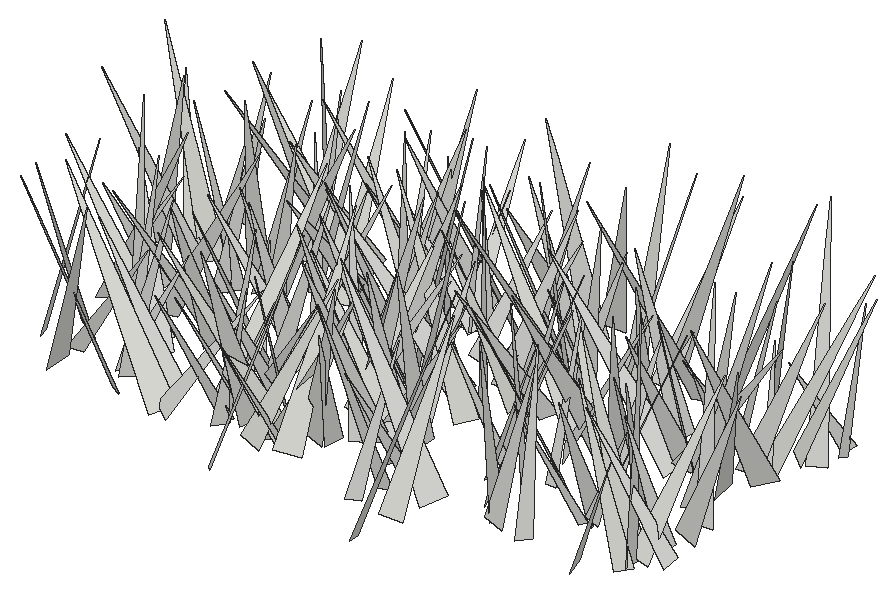
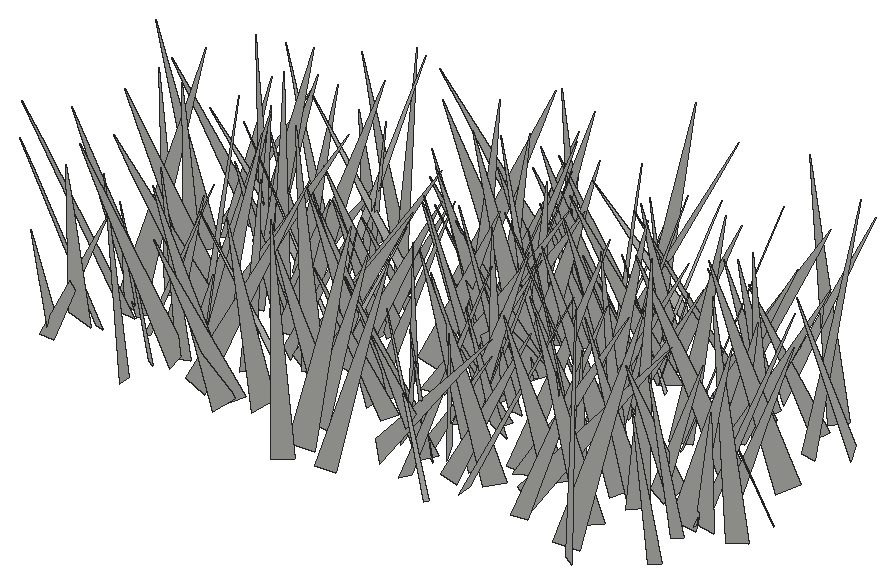
# SketchUp Ruby script. Lengths in inches.
U = 1.inch
M = Sketchup.active_model
def pt(a) = Geom::Point3d.new(a.map { |v| v * U })
def face(e, loops, mat)
  f = e.add_face(loops[0].map { |a| pt(a) })
  loops[1..].each { |l| e.add_face(l.map { |a| pt(a) }).erase! }
  f.material = f.back_material = mat if mat
  f
end
# faces: each face lists its corners as indices into pts; further lists are holes
def faces(e, pts, list, mat = nil) = list.each { |f| face(e, (f[0].is_a?(Array) ? f : [f]).map { |l| l.map { |i| pts[i] } }, mat) }
# xy, xz, yz: faces in a plane at the given z, y or x. An outline is a flat list of corners, or four numbers for a rectangle; further outlines are holes
def ring(l) = l.size == 4 ? [[l[0], l[1]], [l[2], l[1]], [l[2], l[3]], [l[0], l[3]]] : l.each_slice(2).to_a
def flat(e, list, mat, &to3) = list.each { |f| face(e, (f[0].is_a?(Array) ? f : [f]).map { |l| ring(l).map { |u, v| to3.(u, v) } }, mat) }
def xy(e, z, list, mat = nil) = flat(e, list, mat) { |x, y| [x, y, z] }
def xz(e, y, list, mat = nil) = flat(e, list, mat) { |x, z| [x, y, z] }
def yz(e, x, list, mat = nil) = flat(e, list, mat) { |y, z| [x, y, z] }
def lines(e, pts, list) = list.each { |a, b| e.add_line(pt(pts[a]), pt(pts[b])) }
# prism: a flat outline (further loops are holes) pulled along v
def prism(e, loops, v, mat = nil)
  f = face(e, loops, mat); d = Geom::Vector3d.new(v.map { |x| x * U })
  f.pushpull(f.normal.samedirection?(d) ? d.length : -d.length)
end
def box(e, o, s, mat = nil) = prism(e, [[o, [o[0] + s[0], o[1], o[2]], [o[0] + s[0], o[1] + s[1], o[2]], [o[0], o[1] + s[1], o[2]]]], [0, 0, s[2]], mat)
def at(x, y, z, deg = 0) = Geom::Transformation.translation(pt([x, y, z])) * Geom::Transformation.rotation(ORIGIN, Z_AXIS, deg.degrees)
def axes(o, x, y, z) = Geom::Transformation.new([*x, 0, *y, 0, *z, 0, *pt(o).to_a, 1])
def part(name) = M.definitions.add(name)
# library, detail: a bought-in or finely detailed component or shape, given as its bounding box
def library(name, o, s) = part(name).tap { |d| box(d.entities, o, s) }
def detail(e, o, s) = box(e.add_group.entities, o, s)
def put(e, d, t, mat = nil) = e.add_instance(d, t).tap { |i| i.material = mat if mat }
def group(e, t, mat = nil) = e.add_group.tap { |g| g.transformation = t; g.material = mat if mat }.entities
root = M.entities
c1 = part("fur_instance\#9")
p = [[0.8125,0,1.79],[0.67,-0.02,1.48],[0,-0.11,0],[0,0.11,0]]
faces(c1.entities,p,[[0,1,2,3]])
put(root,c1,axes([504.42,389.3125,-21.66],[8.18505,-1.50624,0.16494],[-1.43272,-7.98824,-1.85106],[-0.49323,-1.79175,8.11402]))
put(root,c1,axes([531.82,383.56,-21.66],[7.42778,3.7642,0.92799],[3.25227,-7.14156,2.93652],[-2.11023,2.24305,7.79217]))
put(root,c1,axes([521.25,389.9,-21.66],[-3.70308,-3.24105,0.05421],[-3.08159,3.54543,1.46762],[1.00557,-1.07036,4.69716]))
put(root,c1,axes([518.14,391.06,-21.66],[6.29678,-5.28708,1.00032],[-4.88133,-6.26054,-2.36253],[-2.26416,-1.20654,7.87535]))
put(root,c1,axes([509.29,388.8125,-21.66],[-4.9129,-5.75828,0.52895],[-5.68371,4.68095,-1.83254],[-1.06438,1.58274,7.34412]))
put(root,c1,axes([544.375,389.15,-21.66],[5.4983,0.81734,0.21266],[0.84397,-5.26527,-1.58403],[0.03145,-1.59793,5.32824]))
put(root,c1,axes([520.83,390.58,-21.66],[-8.10416,-1.22815,0.06312],[-1.16757,7.81624,2.17553],[0.38615,-2.14192,7.90272]))
put(root,c1,axes([516.7,390.24,-21.66],[0.11807,-5.18176,0.38422],[-4.95689,-0.22756,-1.54584],[-1.55804,0.33133,4.94722]))
put(root,c1,axes([529.51,389.47,-21.66],[-1.62801,-6.13851,1.48062],[-6.15059,1.19536,-1.80699],[-1.42958,1.84764,6.08822]))
put(root,c1,axes([517.17,391.55,-21.66],[-4.17954,-4.03403,0.06779],[-3.83281,4.00041,1.74723],[1.26,-1.21235,5.53978]))
put(root,c1,axes([532,386.88,-21.66],[-2.25135,6.36064,1.32657],[6.19225,2.52565,-1.60099],[1.96812,-0.67041,6.55463]))
put(root,c1,axes([519.65,384.83,-21.66],[5.70548,5.18554,0.14342],[4.71826,-5.27598,3.06024],[-2.15603,2.1765,7.07653]))
put(root,c1,axes([528.83,387.26,-21.66],[-4.17558,2.72173,1.55923],[2.19552,4.39009,-1.78362],[2.24025,0.77057,4.65424]))
put(root,c1,axes([522.16,391.57,-21.66],[0.1957,-7.90399,1.09327],[-7.43409,0.21668,2.89722],[2.89871,1.0893,7.35646]))
put(root,c1,axes([512.96,388.73,-21.66],[-5.23637,6.32875,0.17784],[5.87309,4.76933,3.20385],[-2.36465,-2.16904,7.5636]))
put(root,c1,axes([513.02,388.52,-21.66],[2.725,5.40327,0.30402],[4.86473,-2.29653,-2.78814],[2.3711,-1.498,5.37096]))
put(root,c1,axes([532.75,390.09,-21.66],[-7.09229,4.18803,1.11711],[4.32642,6.70959,2.31334],[-0.26383,-2.55536,7.90497]))
put(root,c1,axes([536.72,391.13,-21.66],[6.67439,0.3641,2.55328],[0.99441,-6.8993,-1.61558],[-2.3797,-1.86182,6.48614]))
put(root,c1,axes([537.26,390.22,-21.66],[0.1838,-6.38239,2.38865],[-6.46729,0.58989,2.0738],[2.14821,2.32195,6.03888]))
put(root,c1,axes([516.36,390.43,-21.66],[-1.2496,-4.95098,2.04852],[-4.91628,1.89585,1.58307],[2.13046,1.47094,4.85465]))
put(root,c1,axes([519.625,388.79,-21.66],[0.86928,6.52033,1.58307],[6.24969,-0.2059,-2.58369],[2.44176,-1.79425,6.04937]))
put(root,c1,axes([529.21,391.82,-21.66],[1.40326,-4.201,0.43994],[-3.89786,-1.46649,-1.57071],[-1.62745,-0.10993,4.1413]))
put(root,c1,axes([523.49,392.05,-21.66],[4.86782,-2.47433,0.4659],[-2.27673,-4.75873,-1.48527],[-1.07512,-1.1257,5.25471]))
put(root,c1,axes([503.3,393.65,-21.66],[-3.16063,-7.46069,0.64697],[-7.21635,3.22195,1.90087],[2.00118,-0.16476,7.87643]))
put(root,c1,axes([518.74,393.38,-21.66],[-3.46675,-5.54657,1.13696],[-5.08588,3.63649,2.23277],[2.48816,-0.29493,6.14797]))
put(root,c1,axes([511.83,391.42,-21.66],[-4.61226,3.61546,0.79034],[3.61757,4.1381,2.18138],[-0.78062,-2.18488,5.43931]))
put(root,c1,axes([516.79,389.37,-21.66],[-5.68198,1.58826,2.45655],[1.00817,6.10119,-1.61279],[2.74605,1.04639,5.67506]))
put(root,c1,axes([525.66,393.66,-21.66],[3.52912,-6.81057,1.30534],[-6.45742,-3.76145,-2.16695],[-2.52774,0.10047,7.35818]))
put(root,c1,axes([546.97,390.64,-21.66],[-2.40654,5.51072,1.54274],[5.60544,1.9331,1.83892],[-1.15197,-2.10585,5.72519]))
put(root,c1,axes([517.65,394.1,-21.66],[-5.63617,-2.55407,1.20627],[-1.85262,5.37498,2.72438],[2.13217,-2.08115,5.55585]))
put(root,c1,axes([520.44,390.14,-21.66],[6.21247,-1.9108,0.54363],[-1.98453,-5.88708,1.9863],[0.09123,2.05733,6.18874]))
put(root,c1,axes([504.27,391.19,-21.66],[3.95823,-3.37287,0.12226],[-3.1364,-3.60629,2.0534],[1.24667,1.63622,4.7778]))
put(root,c1,axes([539.9,389.82,-21.66],[-5.67085,1.89535,1.35099],[1.57668,5.74544,-1.44226],[1.71219,0.98676,5.80265]))
put(root,c1,axes([507.76,391.4,-21.66],[2.74788,4.31889,0.7575],[4.17328,-2.30167,-2.01583],[1.34551,-1.68135,4.70533]))
put(root,c1,axes([522.2,389.19,-21.66],[-3.86216,7.0455,1.20437],[6.7899,4.04407,-1.88376],[2.2331,-0.11104,7.81068]))
put(root,c1,axes([548.68,393.02,-21.66],[-5.67147,0.82087,0.04901],[0.80443,5.46726,1.5178],[-0.17066,-1.50898,5.5259]))
put(root,c1,axes([508.2,391.07,-21.66],[5.34451,-1.51745,2.02584],[-2.07356,-5.33917,1.4711],[-1.45157,2.03988,5.35746]))
put(root,c1,axes([520.91,391.54,-21.66],[0.51844,5.23573,1.343],[5.13497,-0.0558,-1.76472],[1.68777,-1.43851,4.95655]))
put(root,c1,axes([516.24,391.59,-21.66],[-4.21104,-1.2398,0.43934],[-1.31531,3.95873,-1.43574],[-0.00925,1.50143,4.14832]))
put(root,c1,axes([541.25,395.02,-21.66],[5.27025,-2.47106,0.85487],[-2.00329,-5.05203,-2.25305],[-1.68041,-1.72721,5.36707]))
put(root,c1,axes([514.88,392.86,-21.66],[3.85978,2.30102,0.3483],[2.28006,-3.60384,-1.45862],[0.46617,-1.42533,4.2503]))
put(root,c1,axes([547.47,394.24,-21.66],[-4.78026,1.17069,2.19317],[1.89155,4.79719,1.56216],[1.61324,-2.15588,4.66702]))
put(root,c1,axes([545.3,393.41,-21.66],[3.76435,-5.16952,3.38659],[-5.24976,-4.76711,-1.44149],[-3.26082,1.70703,6.23028]))
put(root,c1,axes([508.73,390.62,-21.66],[-6.51752,1.2418,2.00991],[0.54856,6.53189,-2.25684],[2.29801,1.9627,6.23913]))
put(root,c1,axes([509.04,393.28,-21.66],[-3.24563,2.42896,0.17461],[2.25293,2.88449,1.75171],[-0.92447,-1.49811,3.65588]))
put(root,c1,axes([527.98,395.03,-21.66],[6.98441,-2.34407,2.00985],[-1.86712,-7.16517,-1.86827],[-2.45928,-1.21733,7.12645]))
put(root,c1,axes([541.52,393.58,-21.66],[-1.12844,-4.06047,0.83548],[-3.60524,0.5338,-2.27512],[-2.04639,1.29864,3.54749]))
put(root,c1,axes([546.91,391.41,-21.66],[-7.37531,-1.40171,2.74866],[-2.16749,7.42249,-2.03071],[2.19589,2.61858,7.22747]))
put(root,c1,axes([516.49,393.14,-21.66],[3.7348,-2.45498,0.02516],[-2.33086,-3.53122,1.44009],[0.77113,1.21649,4.23106]))
put(root,c1,axes([537.35,396.87,-21.66],[-4.65731,-6.85842,0.0184],[-6.74044,4.58127,1.51895],[1.26677,-0.83835,8.14992]))
put(root,c1,axes([525.89,395.41,-21.66],[5.91516,-3.3432,1.65321],[-2.9566,-6.09276,-1.74243],[-2.27346,-0.77492,6.56735]))
put(root,c1,axes([509.72,397.79,-21.66],[-6.50454,-4.83681,0.42708],[-4.2184,5.98256,3.50717],[2.40464,-2.5885,7.30777]))
put(root,c1,axes([501.47,391.58,-21.66],[5.51365,3.20537,1.24598],[2.89904,-5.59864,1.57419],[-1.84998,0.77981,6.18035]))
put(root,c1,axes([537.99,392.52,-21.66],[-6.10428,-1.79449,1.71008],[-2.20054,6.01533,-1.54278],[1.14113,2.0006,6.1727]))
put(root,c1,axes([541.73,394.08,-21.66],[0.78956,-4.05986,1.16414],[-3.93825,-0.27989,1.69498],[1.52574,1.37851,3.77266]))
put(root,c1,axes([527.8,392.07,-21.66],[5.78446,0.51407,0.77192],[0.25637,-5.57234,1.78981],[-0.89129,1.73346,5.52457]))
put(root,c1,axes([523.09,395.67,-21.66],[1.43067,-7.01564,1.7352],[-6.90944,-1.84641,-1.76845],[-2.11892,1.28394,6.9382]))
put(root,c1,axes([527.23,393.99,-21.66],[-4.14935,5.21761,0.66717],[4.85978,3.47746,3.02911],[-2.01273,-2.35998,5.93844]))
put(root,c1,axes([510.45,397.01,-21.66],[5.40488,-4.57462,0.50738],[-4.27322,-5.27816,-2.06831],[-1.71004,-1.26929,6.77215]))
put(root,c1,axes([522.02,396.05,-21.66],[7.41722,0.99885,0.34739],[1.05742,-6.96886,-2.53978],[0.01548,-2.56338,7.04006]))
put(root,c1,axes([546.83,392.18,-21.66],[0.07577,6.70614,0.84141],[6.48392,0.16538,-1.90197],[1.90764,-0.82847,6.43122]))
put(root,c1,axes([525.54,394.03,-21.66],[4.06898,-3.86093,0.67624],[-3.71406,-3.48612,2.44405],[1.25293,2.20473,5.04877]))
put(root,c1,axes([525.66,396.5,-21.66],[-7.8024,0.71377,1.7229],[1.19599,7.6017,2.26696],[1.43089,-2.46171,7.49986]))
put(root,c1,axes([507.84,395.1875,-21.66],[-6.653,2.83628,0.09553],[2.75112,6.38619,1.99099],[-0.69638,-1.86767,6.95291]))
put(root,c1,axes([535.25,391.96,-21.66],[6.47525,4.61232,0.40047],[4.47579,-6.41261,1.48613],[-1.18373,0.98374,7.80985]))
put(root,c1,axes([515.37,391.88,-21.66],[-1.37451,8.097,0.63904],[7.82187,1.49419,-2.10823],[2.18815,-0.25501,7.93763]))
put(root,c1,axes([547.38,396.06,-21.66],[1.03631,-6.95808,1.71035],[-6.57848,-0.23906,3.0134],[2.83968,1.98547,6.35675]))
put(root,c1,axes([524.68,393.02,-21.66],[-0.02832,7.80203,1.3013],[7.5934,-0.33756,2.1891],[-2.2148,-1.25708,7.48868]))
put(root,c1,axes([507.48,392.99,-21.66],[-7.86516,0.65945,1.92725],[0.13584,7.83978,-2.12819],[2.03241,2.02799,7.60042]))
put(root,c1,axes([533.8125,395.94,-21.66],[-0.35504,-4.51922,1.36303],[-4.31721,-0.2418,-1.92625],[-1.90863,1.3876,4.10353]))
put(root,c1,axes([515.41,396.2,-21.66],[-2.41735,-5.08882,0.8159],[-4.81582,1.90935,-2.35956],[-1.83565,1.69223,5.11586]))
put(root,c1,axes([508.69,394.14,-21.66],[-2.09774,5.99421,0.07606],[5.73274,1.98235,1.88224],[-1.75272,-0.69034,6.06533]))
put(root,c1,axes([533.58,394.26,-21.66],[3.9731,1.20771,1.01378],[0.70264,-3.81635,1.79266],[-1.41159,1.49959,3.74573]))
put(root,c1,axes([515.65,398.16,-21.66],[3.87648,-5.20572,1.47803],[-5.00062,-4.14086,-1.46909],[-2.0683,0.2548,6.32205]))
put(root,c1,axes([541.99,398.25,-21.66],[-0.85203,-5.57664,0.61964],[-5.3803,0.98986,1.51043],[1.59225,0.36067,5.43539]))
put(root,c1,axes([542.01,393.95,-21.66],[5.76242,3.50846,0.12226],[3.39302,-5.62636,1.53663],[-0.90093,1.2508,6.56914]))
put(root,c1,axes([516.08,395.29,-21.66],[6.10707,-2.19869,2.10682],[-2.76305,-5.98564,1.76265],[-1.28003,2.43046,6.24689]))
put(root,c1,axes([522.17,396.5625,-21.66],[6.94828,-4.27135,1.74082],[-4.55894,-6.83788,1.41876],[-0.70067,2.13364,8.03182]))
put(root,c1,axes([516.23,398.31,-21.66],[-6.42762,0.7775,0.36666],[0.8533,6.10569,2.01137],[0.10407,-2.04186,6.15412]))
put(root,c1,axes([526.8125,395.1,-21.66],[7.21368,2.51232,2.17903],[2.05011,-7.45745,1.81123],[-2.61859,1.08246,7.42081]))
put(root,c1,axes([526.13,397.39,-21.66],[-3.48224,-3.77241,0.29956],[-3.58403,3.15695,-1.90663],[-1.21472,1.49981,4.76674]))
put(root,c1,axes([537.04,401.39,-21.66],[4.97759,-6.71856,0.2944],[-6.18791,-4.7191,-3.07278],[-2.63353,-1.61035,7.77647]))
put(root,c1,axes([501.76,397.46,-21.66],[6.68383,-3.60485,0.36068],[-3.59385,-6.50181,1.61538],[0.45749,1.59067,7.42019]))
put(root,c1,axes([539.02,399.87,-21.66],[7.15666,-2.1147,0.99823],[-1.83229,-7.06792,-1.83669],[-1.45298,-1.50292,7.233]))
put(root,c1,axes([514.55,396.09,-21.66],[0.6459,3.9486,0.07217],[3.68247,-0.62859,1.43463],[-1.42692,0.16515,3.73504]))
put(root,c1,axes([540.52,400.16,-21.66],[-1.15105,-5.30671,0.17],[-5.09537,1.15297,1.49093],[1.49242,-0.15644,5.22142]))
put(root,c1,axes([532.19,397.24,-21.66],[5.41003,-2.25588,0.78895],[-2.38957,-5.13634,1.69936],[-0.03699,1.87321,5.60977]))
put(root,c1,axes([522.25,395.64,-21.66],[-1.13308,6.40977,0.66119],[6.08836,1.28481,-2.02171],[2.11049,-0.26515,6.18722]))
put(root,c1,axes([526.18,397,-21.66],[-0.72846,5.64896,1.65026],[5.62241,1.15927,-1.48642],[1.73859,-1.38206,5.49837]))
put(root,c1,axes([503.7,400.38,-21.66],[3.91388,-2.85851,1.41513],[-2.09693,-3.9939,-2.26798],[-2.40345,-1.17037,4.2832]))
put(root,c1,axes([537.02,396.01,-21.66],[1.91748,5.33638,0.31642],[5.10909,-1.9283,1.55969],[-1.57297,0.24194,5.4517]))
put(root,c1,axes([505.78,397.99,-21.66],[5.9864,-4.39629,0.74457],[-4.35138,-5.48795,2.58196],[0.97326,2.50473,6.96403]))
put(root,c1,axes([522.33,401.29,-21.66],[-7.22673,-3.69522,1.05519],[-3.3656,7.17065,2.06111],[1.85494,-1.38592,7.85061]))
put(root,c1,axes([521.2,398.23,-21.66],[4.19059,5.13354,0.34706],[4.85008,-3.79176,-2.47669],[1.71767,-1.81771,6.14657]))
put(root,c1,axes([525.96,401.47,-21.66],[-7.44265,2.94787,0.75024],[2.95668,6.54484,3.6151],[-0.71474,-3.62229,7.14241]))
put(root,c1,axes([535.19,399.57,-21.66],[5.77692,4.11347,0.10405],[3.90568,-5.42514,-2.37018],[1.29504,-1.98782,6.68399]))
put(root,c1,axes([545.58,401.95,-21.66],[6.93671,-0.62868,0.23505],[-0.51232,-6.5363,-2.3628],[-0.4336,-2.33453,6.55213]))
put(root,c1,axes([547.41,397.8,-21.66],[1.24745,7.40868,1.63783],[7.39275,-1.56046,1.42803],[-1.70827,-1.34297,7.376]))
put(root,c1,axes([515.06,399.18,-21.66],[5.08074,5.57509,0.64514],[5.46993,-4.72427,-2.25231],[1.25607,-1.97773,7.19879]))
put(root,c1,axes([532.65,398.03,-21.66],[5.29795,0.17393,1.896],[-0.4687,-5.31448,1.7972],[-1.84537,1.84915,4.98684]))
put(root,c1,axes([531.67,402.59,-21.66],[2.44843,-5.51273,0.60157],[-4.8536,-2.44839,-2.68234],[-2.6823,-0.60174,5.40279]))
put(root,c1,axes([521.76,399.03,-21.66],[6.06814,-4.77445,2.10475],[-5.2154,-5.64781,2.22478],[-0.15808,3.05854,7.39379]))
put(root,c1,axes([541.93,403.08,-21.66],[4.15216,-5.25606,0.30062],[-4.95254,-4.0295,-2.04756],[-1.78575,-1.04593,6.37763]))
put(root,c1,axes([528.15,398.97,-21.66],[-2.68904,7.46116,1.26428],[7.06219,1.99214,3.26422],[-2.71897,-2.20471,7.22805]))
put(root,c1,axes([539.2,399.55,-21.66],[-0.86303,4.80618,1.97762],[4.83833,1.47497,-1.47315],[1.8976,-1.57489,4.65553]))
put(root,c1,axes([512.11,401.82,-21.66],[-5.24413,-0.63684,1.6828],[-0.10679,5.28634,1.66778],[1.7961,-1.54509,5.01248]))
put(root,c1,axes([546.99,404.26,-21.66],[4.52461,-6.7861,0.00105],[-6.53347,-4.35651,-2.20405],[-1.83437,-1.22185,7.85273]))
put(root,c1,axes([539.01,399.04,-21.66],[-2.13966,5.92839,0.3544],[5.56639,1.87053,2.31645],[-2.07043,-1.09766,5.86157]))
put(root,c1,axes([542.28,403.04,-21.66],[-3.66849,-5.82093,1.22872],[-5.44278,3.86666,2.06783],[2.40191,-0.1285,6.56241]))
put(root,c1,axes([541.65,402.26,-21.66],[-7.78216,2.50032,0.23977],[2.4235,7.26917,2.85602],[-0.66011,-2.78901,7.65877]))
put(root,c1,axes([529.37,402.27,-21.66],[-6.5147,0.26004,1.16019],[0.55336,6.38259,1.67669],[1.05235,-1.74639,6.3006]))
put(root,c1,axes([520.51,400.36,-21.66],[2.74298,6.25055,1.8619],[6.47418,-2.36552,-1.59662],[0.78801,-2.32269,6.63657]))
put(root,c1,axes([516,405.83,-21.66],[6.60243,-3.6292,1.16999],[-2.40466,-5.77841,-4.35427],[-2.95933,-3.40161,6.14845]))
put(root,c1,axes([510.49,402.54,-21.66],[0.32033,-6.88611,1.90206],[-6.92731,0.16595,1.76741],[1.74605,1.92169,6.66313]))
put(root,c1,axes([499.67,401.52,-21.66],[3.27011,3.05252,0.13659],[2.8317,-2.95233,-1.81533],[1.14804,-1.41282,4.08853]))
put(root,c1,axes([534.22,403.875,-21.66],[-2.23996,-8.03771,0.28468],[-7.44594,1.96073,-3.22749],[-3.04036,1.11981,7.69451]))
put(root,c1,axes([503.21,404.1,-21.66],[-7.55604,-1.18176,1.01335],[-0.88861,7.39753,2.00103],[1.27821,-1.84315,7.38147]))
put(root,c1,axes([514.61,400.91,-21.66],[4.76351,-2.22786,1.63166],[-2.67424,-4.53288,1.61806],[-0.68857,2.19233,5.00362]))
put(root,c1,axes([545.27,399.24,-21.66],[7.73551,0.03019,2.73159],[-1.01366,-7.58581,2.95441],[-2.53672,3.12332,7.14916]))
put(root,c1,axes([522.16,400.19,-21.66],[-7.61718,0.0241,1.98426],[-0.51537,7.57673,-2.07045],[1.91631,2.1335,7.33043]))
put(root,c1,axes([519.91,401.76,-21.66],[0.48143,3.7055,0.846],[3.27794,0.02687,-1.98307],[1.92393,-0.97302,3.16701]))
put(root,c1,axes([522.75,400.45,-21.66],[7.20277,3.49638,1.97973],[3.12762,-7.42996,1.74287],[-2.5223,0.77133,7.81454]))
put(root,c1,axes([535.77,403.24,-21.66],[-2.3451,-4.39084,0.71964],[-4.31416,2.04482,-1.58228],[-1.08875,1.35503,4.71968]))
put(root,c1,axes([534.6,401.77,-21.66],[-4.02573,7.19257,0.41274],[6.48293,3.4104,3.80141],[-3.14246,-2.17854,7.31361]))
put(root,c1,axes([541.81,402.59,-21.66],[4.55,-4.60588,0.41001],[-4.16176,-3.82822,3.1795],[2.01545,2.49305,5.6398]))
put(root,c1,axes([533.07,404.09,-21.66],[0.67729,-7.55263,2.0847],[-7.70125,-0.25666,1.57216],[1.44182,2.17688,7.41817]))
put(root,c1,axes([507.36,405.01,-21.66],[7.0973,-2.99001,1.53723],[-2.6894,-7.20395,-1.59536],[-2.01752,-0.91535,7.53436]))
put(root,c1,axes([521.97,403.39,-21.66],[-5.92654,3.46188,1.28835],[3.68281,5.72588,1.55549],[0.28525,-1.99951,6.68498]))
put(root,c1,axes([500.04,404.54,-21.66],[1.15039,-7.47242,1.55869],[-7.41634,-0.72104,2.01691],[1.80677,1.79806,7.28646]))
put(root,c1,axes([527.53,401.36,-21.66],[-6.50203,-1.48304,1.94789],[-2.15091,6.10063,-2.53495],[1.1693,2.97539,6.16846]))
put(root,c1,axes([509.24,403.95,-21.66],[5.85705,-5.48153,0.51052],[-5.36351,-5.5136,2.33363],[1.24121,2.04104,7.67505]))
put(root,c1,axes([507.39,403.05,-21.66],[-2.16703,-5.16397,2.37315],[-5.48971,1.24499,-2.30381],[-1.47021,2.96275,5.10441]))
put(root,c1,axes([542.55,406.16,-21.66],[3.43107,-2.8474,0.0502],[-2.64084,-3.2106,-1.6126],[-1.06592,-1.21113,4.15686]))
put(root,c1,axes([543.73,406.72,-21.66],[-4.54437,-2.07997,0.71062],[-1.49312,4.11891,2.50752],[1.61302,-2.04715,4.32318]))
put(root,c1,axes([539.58,405.6,-21.66],[-6.14349,2.42883,3.06477],[3.31416,6.26335,1.67969],[2.07568,-2.81172,6.38908]))
put(root,c1,axes([511.83,404.69,-21.66],[6.05057,5.41917,1.99571],[5.77348,-5.74186,-1.9125],[-0.1309,-2.76104,7.89425]))
put(root,c1,axes([536.23,406.39,-21.66],[5.5268,-1.95543,1.04999],[-1.67194,-5.52102,-1.48142],[-1.45972,-1.07995,5.67227]))
put(root,c1,axes([527.36,403.54,-21.66],[-2.26569,5.88907,2.62757],[5.5866,3.18358,-2.31806],[3.22106,-1.37923,5.86866]))
put(root,c1,axes([513.45,403.06,-21.66],[-5.70107,0.73605,0.76728],[0.48907,5.53142,-1.67238],[0.94409,1.57933,5.49974]))
put(root,c1,axes([508.53,403.69,-21.66],[6.30569,-0.68619,2.05979],[-1.17683,-6.39727,1.4715],[-1.82446,1.75482,6.16987]))
put(root,c1,axes([531.38,405.74,-21.66],[-5.94217,-4.1756,0.21971],[-4.13273,5.80684,-1.41225],[-0.63601,1.27993,7.12394]))
put(root,c1,axes([545.28,404.69,-21.66],[4.70932,-5.02611,1.74089],[-5.27526,-4.11549,2.38842],[0.68127,2.87596,6.46026]))
put(root,c1,axes([506.62,402.16,-21.66],[-6.46453,1.71895,1.7422],[0.79023,6.12289,-3.109],[2.31637,2.70842,5.92275]))
put(root,c1,axes([532.46,403.85,-21.66],[-6.42625,-2.81034,1.42452],[-3.14557,5.90814,-2.53441],[0.18076,2.90169,6.53999]))
put(root,c1,axes([503.95,404.875,-21.66],[-2.60972,7.0339,1.93347],[7.14895,2.0575,2.16424],[-1.45142,-2.51309,7.18348]))
put(root,c1,axes([515.29,405.94,-21.66],[-6.72983,3.60579,0.05795],[3.45053,6.40273,2.3226],[-1.04828,-2.07339,7.27309]))
put(root,c1,axes([503.29,406.28,-21.66],[0.14432,-5.01914,1.5992],[-4.96199,0.40759,1.72702],[1.76858,1.55311,4.71487]))
put(root,c1,axes([519.85,402.77,-21.66],[1.21236,6.8418,0.01969],[6.58716,-1.17263,1.87473],[-1.84929,0.30844,6.6907]))
put(root,c1,axes([527.87,404.34,-21.66],[7.54644,-1.30772,2.23251],[-1.88035,-7.50036,1.96263],[-1.77721,2.38276,7.40318]))
put(root,c1,axes([502.68,404.39,-21.66],[-0.8171,5.77252,0.59098],[5.63961,0.64951,1.4532],[-1.36602,-0.77139,5.64605]))
put(root,c1,axes([531.01,405.7,-21.66],[4.31663,-3.25233,1.38409],[-3.53279,-4.03972,1.52536],[-0.11299,2.05661,5.185]))
put(root,c1,axes([525.99,405.57,-21.66],[3.23121,-4.00646,1.7311],[-4.24322,-2.37965,2.41277],[1.02152,2.78831,4.54653]))
put(root,c1,axes([513.48,408.17,-21.66],[-2.19661,-7.3796,0.4517],[-6.30745,1.62463,-4.13089],[-3.85727,1.54587,6.49764]))
put(root,c1,axes([546.67,404.73,-21.66],[0.48963,4.22721,0.04806],[3.94805,-0.47454,1.51627],[-1.51146,0.12987,3.97618]))
put(root,c1,axes([512.29,410.24,-21.66],[6.08199,-2.63161,2.26399],[-1.13407,-5.82276,-3.72169],[-3.281,-2.8656,5.48316]))
put(root,c1,axes([524,405.27,-21.66],[-0.28996,5.60424,1.15409],[5.32871,0.68543,-1.98963],[2.08431,-0.97272,5.24719]))
put(root,c1,axes([540.14,407.72,-21.66],[-0.32261,-5.78503,1.74562],[-5.69921,0.87225,1.8374],[2.00818,1.5461,5.49497]))
put(root,c1,axes([546.14,405.6,-21.66],[3.48936,7.09192,0.65775],[6.9322,-3.21357,-2.12629],[1.63479,-1.51038,7.61247]))
put(root,c1,axes([518.51,409.26,-21.66],[0.56796,-5.36738,0.34113],[-5.01782,-0.65229,-1.90884],[-1.93561,0.11605,5.04853]))
put(root,c1,axes([521.62,408.03,-21.66],[-4.01783,2.35497,0.3103],[2.27352,3.63609,1.84258],[-0.68795,-1.73727,4.27712]))
put(root,c1,axes([537.57,409.85,-21.66],[-1.57704,-7.74459,0.50786],[-7.45096,1.36569,-2.31124],[-2.17253,0.93802,7.55804]))
put(root,c1,axes([516.91,409.73,-21.66],[-7.35388,-1.92649,0.06127],[-1.88282,7.23164,1.39751],[0.41243,-1.33667,7.47248]))
put(root,c1,axes([513.2,405.53,-21.66],[-3.83392,6.10516,1.11787],[5.9137,3.99214,-1.52073],[1.88436,-0.10697,7.04694]))
put(root,c1,axes([520.8125,410.6,-21.66],[-7.04471,-1.4589,1.32068],[-0.96261,6.83613,2.41686],[1.71638,-2.15394,6.77607]))
put(root,c1,axes([520.48,406.74,-21.66],[-5.01766,-1.40088,1.70753],[-1.93126,4.83928,-1.7049],[1.07162,2.16194,4.92267]))
put(root,c1,axes([511.08,405.79,-21.66],[-5.97598,0.81352,1.54005],[0.17172,5.75229,-2.37225],[1.73323,2.235,5.54496]))
put(root,c1,axes([517.9375,406.8125,-21.66],[7.25129,-2.23194,2.73946],[-2.93898,-7.28136,1.84704],[-1.96177,2.6585,7.35875]))
put(root,c1,axes([515.91,408.07,-21.66],[3.27115,-5.93629,2.22387],[-6.24966,-2.60094,2.25],[1.06155,2.98013,6.39355]))
put(root,c1,axes([528.81,409.09,-21.66],[1.01091,-5.94061,2.30759],[-6.04054,-1.63799,-1.57056],[-2.03168,1.91413,5.81775]))
put(root,c1,axes([507.83,411.25,-21.66],[3.07442,-7.15508,0.96712],[-6.88437,-3.22185,-1.95131],[-2.1762,0.08396,7.5392]))
put(root,c1,axes([546.61,407.8,-21.66],[3.72746,5.46093,0.78491],[5.42353,-3.45332,-1.72965],[1.01153,-1.60767,6.38153]))
put(root,c1,axes([534.61,405.1875,-21.66],[5.37795,5.75,0.47067],[5.40496,-5.24661,2.33794],[-2.01755,1.27162,7.51791]))
put(root,c1,axes([548.32,410.7,-21.66],[2.70067,-3.13661,0.88183],[-2.51329,-2.73437,-2.02883],[-2.07348,-0.77102,3.60774]))
put(root,c1,axes([523.68,406.97,-21.66],[-4.92435,-0.05312,0.24709],[-0.15186,4.47527,-2.06445],[0.20202,2.06935,4.47102]))
put(root,c1,axes([502.33,409.64,-21.66],[0.76926,-4.66703,1.07076],[-4.59745,-0.41678,1.48633],[1.33832,1.25083,4.49041]))
put(root,c1,axes([541.43,409.33,-21.66],[3.4231,3.63538,1.50249],[3.93251,-3.11512,-1.42212],[0.09387,-2.06666,4.78656]))
put(root,c1,axes([525.06,412.96,-21.66],[5.40671,-4.03304,0.21931],[-3.53675,-4.90438,-2.9974],[-1.95061,-2.2864,6.04264]))
put(root,c1,axes([521.23,407.73,-21.66],[2.56304,5.03632,1.18387],[4.82189,-2.80423,1.49027],[-1.87495,-0.32715,5.45094]))
put(root,c1,axes([508.32,408.29,-21.66],[-2.56408,6.91655,2.55207],[6.94878,3.17004,-1.60986],[2.46298,-1.74312,7.19872]))
put(root,c1,axes([524.03,409.2,-21.66],[-5.38862,-5.55187,0.24968],[-4.68183,4.34761,-4.37054],[-2.99434,3.19341,6.38427]))
put(root,c1,axes([540.44,407.97,-21.66],[8.13769,0.92636,1.08085],[0.65484,-8.00564,1.93114],[-1.26395,1.81658,7.95932]))
put(root,c1,axes([517.89,412.1875,-21.66],[5.66121,2.03663,0.41958],[1.99596,-4.98096,-2.75306],[0.58316,-2.72311,5.34956]))
put(root,c1,axes([521.08,407.99,-21.66],[-3.49002,4.97532,0.38419],[4.70613,3.43753,-1.76559],[1.65943,0.71499,5.81522]))
put(root,c1,axes([527.9,411.73,-21.66],[2.50523,-6.92108,2.84903],[-7.08461,-3.16179,-1.45116],[-2.41383,2.09672,7.21607]))
put(root,c1,axes([548.07,407.84,-21.66],[0.30584,8.28043,0.48557],[7.987,-0.4251,2.21855],[-2.2381,-0.38549,7.98355]))
put(root,c1,axes([541.33,411.98,-21.66],[6.22131,1.299,1.34326],[1.60809,-6.10017,-1.54868],[-0.95174,-1.81575,6.1639]))
put(root,c1,axes([506.64,412.55,-21.66],[-4.19902,-6.23031,2.61813],[-6.01537,4.8505,1.89504],[3.08005,0.97931,7.27031]))
put(root,c1,axes([532.84,409.22,-21.66],[-6.71814,2.72987,2.53139],[2.23652,7.13443,-1.75826],[2.97626,0.8008,7.03521]))
put(root,c1,axes([527.91,413.51,-21.66],[2.36593,-6.95857,0.28973],[-6.83072,-2.25873,1.53056],[1.359,0.76137,7.18865]))
put(root,c1,axes([548.5625,409.76,-21.66],[-4.5247,0.14497,1.56827],[-0.47946,4.4174,-1.79167],[1.5002,1.84904,4.15738]))
put(root,c1,axes([534.73,410.65,-21.66],[7.47756,-1.51643,1.55812],[-1.8154,-7.42558,1.48539],[-1.19651,1.78955,7.48379]))
put(root,c1,axes([534.61,409.76,-21.66],[-3.66435,5.27166,1.90181],[4.6134,4.12758,-2.55233],[3.18179,0.08644,5.89097]))
